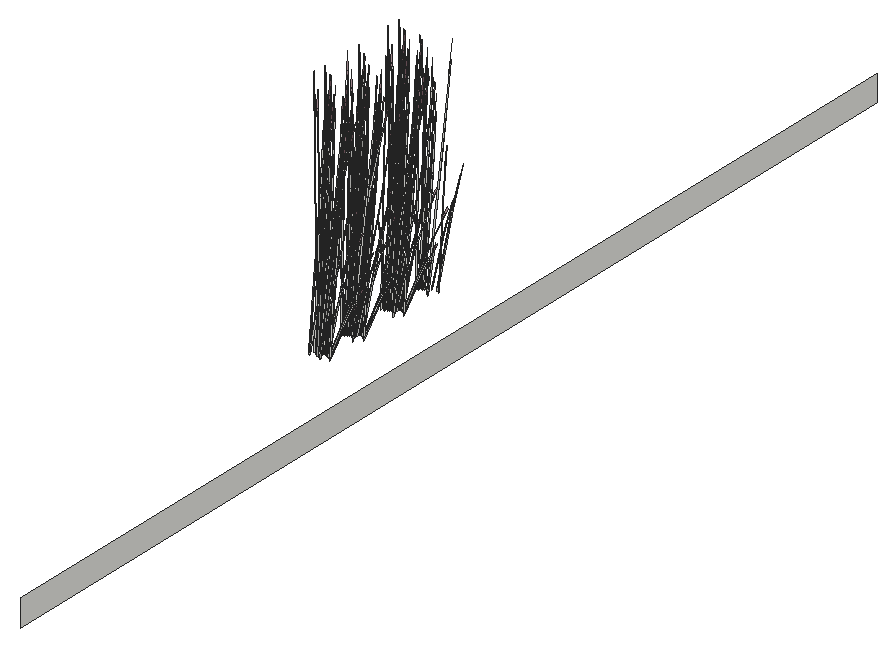
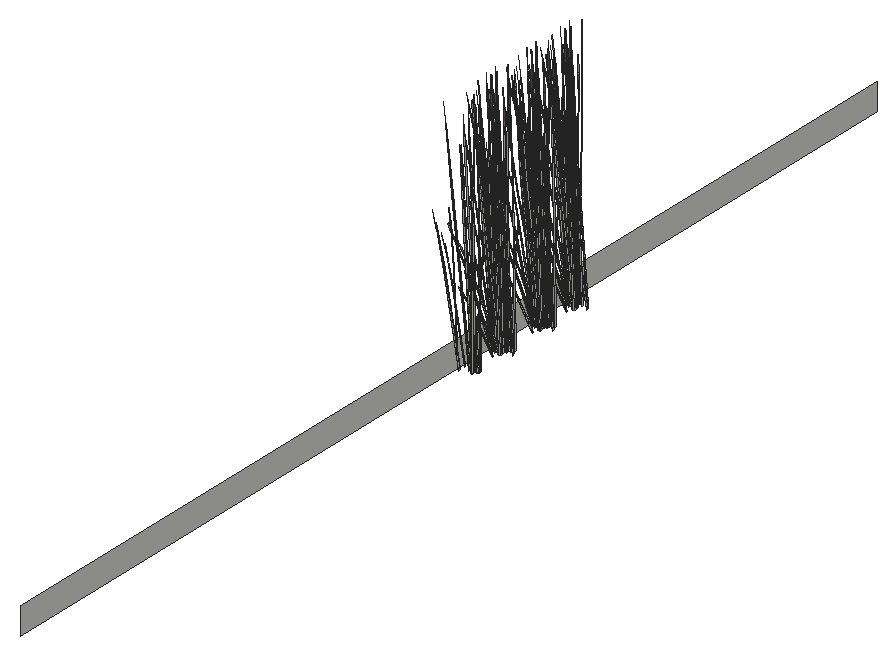
# SketchUp Ruby script. Lengths in inches.
U = 1.inch
M = Sketchup.active_model
def pt(a) = Geom::Point3d.new(a.map { |v| v * U })
def face(e, loops, mat)
  f = e.add_face(loops[0].map { |a| pt(a) })
  loops[1..].each { |l| e.add_face(l.map { |a| pt(a) }).erase! }
  f.material = f.back_material = mat if mat
  f
end
# faces: each face lists its corners as indices into pts; further lists are holes
def faces(e, pts, list, mat = nil) = list.each { |f| face(e, (f[0].is_a?(Array) ? f : [f]).map { |l| l.map { |i| pts[i] } }, mat) }
# xy, xz, yz: faces in a plane at the given z, y or x. An outline is a flat list of corners, or four numbers for a rectangle; further outlines are holes
def ring(l) = l.size == 4 ? [[l[0], l[1]], [l[2], l[1]], [l[2], l[3]], [l[0], l[3]]] : l.each_slice(2).to_a
def flat(e, list, mat, &to3) = list.each { |f| face(e, (f[0].is_a?(Array) ? f : [f]).map { |l| ring(l).map { |u, v| to3.(u, v) } }, mat) }
def xy(e, z, list, mat = nil) = flat(e, list, mat) { |x, y| [x, y, z] }
def xz(e, y, list, mat = nil) = flat(e, list, mat) { |x, z| [x, y, z] }
def yz(e, x, list, mat = nil) = flat(e, list, mat) { |y, z| [x, y, z] }
def lines(e, pts, list) = list.each { |a, b| e.add_line(pt(pts[a]), pt(pts[b])) }
# prism: a flat outline (further loops are holes) pulled along v
def prism(e, loops, v, mat = nil)
  f = face(e, loops, mat); d = Geom::Vector3d.new(v.map { |x| x * U })
  f.pushpull(f.normal.samedirection?(d) ? d.length : -d.length)
end
def box(e, o, s, mat = nil) = prism(e, [[o, [o[0] + s[0], o[1], o[2]], [o[0] + s[0], o[1] + s[1], o[2]], [o[0], o[1] + s[1], o[2]]]], [0, 0, s[2]], mat)
def at(x, y, z, deg = 0) = Geom::Transformation.translation(pt([x, y, z])) * Geom::Transformation.rotation(ORIGIN, Z_AXIS, deg.degrees)
def axes(o, x, y, z) = Geom::Transformation.new([*x, 0, *y, 0, *z, 0, *pt(o).to_a, 1])
def part(name) = M.definitions.add(name)
# library, detail: a bought-in or finely detailed component or shape, given as its bounding box
def library(name, o, s) = part(name).tap { |d| box(d.entities, o, s) }
def detail(e, o, s) = box(e.add_group.entities, o, s)
def put(e, d, t, mat = nil) = e.add_instance(d, t).tap { |i| i.material = mat if mat }
def group(e, t, mat = nil) = e.add_group.tap { |g| g.transformation = t; g.material = mat if mat }.entities
root = M.entities
M.materials.add("LightPink_Translucent").color = [144, 107, 117]
M.materials["LightPink_Translucent"].alpha = 0.75
c1 = part("blade")
p = [[2.15,0.21,22],[0,0.17,0],[0.09,0.45,0],[2.18,0.31,22],[2.29,0.31,22],[0.38,0.45,0],
  [2.48,0.24,33],[2.49,0.24,33],[2.48,0.22,33]]
faces(c1.entities,p,[[0,1,2,3],[4,5,2,3],[6,3,4,7],[8,0,3,6]])
c2 = part("seeds")
p = [[0.3,-0.1,1.38],[-0.01,-0.03,1.59],[-0.01,-0.03,0.03],[0.14,-0.07,-0.07],[0.29,-0.03,3],[0.15,0.01,3.11]]
faces(c2.entities,p,[[0,1,2,3],[1,0,4,5]],"LightPink_Translucent")
c3 = part("blade with seeds")
put(c3.entities,c1,at(0,0,0))
put(c3.entities,c2,axes([2.4,0.25,30.99],[1.5799,-0.05474,1.17369],[-0.12525,1.92788,0.29478],[-0.07173,-0.02425,1.56792]))
yz(root,346,[[268,42,508,48]])
put(root,c3,axes([335.24,364.91,50.1],[0.31568,-0.39156,0],[0.52815,0.21836,-0.456],[0.12029,0.04973,1.44655]))
put(root,c3,axes([336.49,366.46,49.75],[-0.3252,0.04689,1.25103],[-0.05176,-0.37326,0.07161],[0.22777,-0.0565,0.71188]))
put(root,c3,axes([337.08,366.125,50],[-0.31304,-0.24986,-0.05733],[0.34284,-0.22894,-0.25992],[0.09714,-0.01612,0.85731]))
put(root,c3,axes([334.21,366.16,49.95],[0,-0.45213,0],[0.63136,0,0],[0,0,1.58567]))
put(root,c3,axes([334.97,365.11,50.19],[-0.47255,-0.19538,0.43871],[0.28245,-0.35034,0],[0.10763,0.0445,1.3917]))
put(root,c3,axes([333.91,365.87,50.09],[-0.41865,0.35461,0.40429],[-0.49737,-0.31303,0.15865],[0.10093,-0.03539,1.40366]))
put(root,c3,axes([333.18,365.29,50.1875],[-0.14586,0.38834,0.15589],[-0.53375,-0.1099,0.31002],[0.0922,-0.00189,1.41735]))
put(root,c3,axes([332.96,365.6,49.41],[-0.49699,0.15644,1.13921],[-0.15819,-0.44887,0.44265],[0.30518,0.00747,1.29573]))
put(root,c3,axes([334.29,365.72,50.3125],[0.09741,-0.34873,0.12794],[0.4759,0.06053,-0.36534],[0.08661,0.03581,1.11991]))
put(root,c3,axes([336.84,366.21,49.32],[-0.02639,-0.05932,1.55816],[0.18302,-0.34702,-0.23804],[0.18462,-0.00499,0.26541]))
put(root,c3,axes([334.09,365.8125,50.4],[-0.30332,-0.32798,0.39531],[0.45944,-0.23096,-0.19025],[0.09816,0.04058,1.26923]))
put(root,c3,axes([334.25,365.83,50.36],[0.50979,-0.25942,-0.25709],[0.339,0.36656,-0.44182],[0.12578,0.03723,1.41118]))
put(root,c3,axes([335.53,365.14,49.78],[0.47255,0.19538,-0.43871],[-0.28245,0.35034,0],[0.10763,0.0445,1.3917]))
put(root,c3,axes([334.63,366.26,49.95],[0.56491,0,0],[0,0.40454,0],[0,0,1.5764]))
put(root,c3,axes([334.79,365.31,50.1875],[-0.54257,0.10371,0.15589],[-0.13397,-0.38597,0.31002],[0.04839,0.05624,1.41735]))
put(root,c3,axes([335.4,365.29,49.79],[0.11861,0.34048,-0.27372],[-0.47106,0.09668,0.27372],[0.09497,0.03926,1.22797]))
put(root,c3,axes([334.45,366.05,50.1],[-0.63817,-0.08233,0.43472],[0.12987,-0.46497,0.17059],[0.09326,0.0449,1.50931]))
put(root,c3,axes([334.56,367.15,49.93],[0.53009,-0.13258,-0.16963],[0.18627,0.38191,0.00007],[0.05851,-0.01465,1.53656]))
put(root,c3,axes([334.62,366.43,49.96],[0.35245,0.2524,0],[-0.35245,0.2524,0],[0,0,1.49564]))
put(root,c3,axes([335.58,366.32,50.1875],[-0.39671,-0.28463,0.15589],[0.39978,-0.27607,0.31002],[-0.04381,0.05813,1.41735]))
put(root,c3,axes([334.84,365.89,49.82],[0.52523,0.06406,-0.55095],[-0.11084,0.39517,-0.1446],[0.15674,0.04788,1.21613]))
put(root,c3,axes([334.62,366.14,50.4],[0.24498,-0.3521,0.39531],[0.50902,0.16945,-0.19025],[0,0.08116,1.26923]))
put(root,c3,axes([334.52,366.34,50.03],[0,0.45191,-0.04981],[-0.63136,0,0],[0,0.0142,1.58489]))
put(root,c3,axes([334.57,366.02,49.95],[0.30332,0.32798,-0.39531],[-0.45944,0.23096,0.19025],[0.09816,0.04058,1.26923]))
put(root,c3,axes([335.9,366.33,50.19],[0,-0.39075,0.43871],[0.56491,0,0],[0,0.089,1.3917]))
put(root,c3,axes([334.83,366.22,50.3125],[0.47043,-0.11396,0.12794],[0.16474,0.32541,-0.36534],[0,0.07162,1.11991]))
put(root,c3,axes([336.58,367.01,50.29],[-0.1216,-0.0961,1.26356],[0.15822,-0.31792,-0.27174],[0.24603,0.04307,0.54024]))
put(root,c3,axes([334.4,367.36,49.95],[0.50902,0.17543,0],[-0.24498,0.36452,0],[0,0,1.54589]))
put(root,c3,axes([334.22,367.21,50.02],[0.21952,0.44891,-0.05313],[-0.62724,0.1573,0],[0.00767,0.01568,1.52132]))
put(root,c3,axes([336.29,366.4,50.1],[0.63136,0,0],[0,0.43672,-0.456],[0,0.09947,1.44655]))
put(root,c3,axes([336.03,366.625,49.94],[-0.63105,-0.00312,-0.04397],[0,-0.43672,0.44129],[-0.01983,0.09942,1.3992]))
put(root,c3,axes([334.67,366.24,50.36],[0.56863,0.18645,-0.25709],[-0.2738,0.39352,-0.44182],[0.01787,0.09662,1.41118]))
put(root,c3,axes([335.9,366.6875,49.79],[-0.35245,0.2438,-0.27372],[-0.35245,-0.2438,0.27372],[0,0.07853,1.22797]))
put(root,c3,axes([336.15,366.7,49.78],[0,0.39075,-0.43871],[-0.56491,0,0],[0,0.089,1.3917]))
put(root,c3,axes([335.51,367.92,49.32],[0.03679,-0.05641,1.55816],[0.46313,-0.16615,-0.23804],[0.14041,0.08599,0.26541]))
put(root,c3,axes([334.9,366.64,49.85],[0.18514,0.35777,-0.61156],[-0.53331,0.12885,-0.16051],[0.02046,0.12115,1.3499]))
put(root,c3,axes([335.47,368.02,50.36],[-0.32378,-0.01225,0.92831],[0.21383,-0.26028,0.51254],[0.12791,0.09247,0.72818]))
put(root,c3,axes([334.42,367.39,50.29],[0.00891,-0.12953,1.26356],[0.4258,-0.14469,-0.27174],[0.13144,0.15503,0.54024]))
put(root,c3,axes([334.77,373.97,50.29],[-0.14352,0.07909,1.26356],[-0.42983,-0.13843,-0.27174],[0.07968,-0.17216,0.54024]))
put(root,c3,axes([335.77,374.21,49.32],[-0.07557,-0.03078,1.55816],[-0.19412,-0.34391,-0.23804],[0.13095,-0.09333,0.26541]))
put(root,c3,axes([332.92,374.28,50.1],[-0.31568,-0.39156,0],[0.52815,-0.21836,-0.456],[0.12029,-0.04973,1.44655]))
put(root,c3,axes([333.35,374.22,49.78],[0.47255,-0.19538,-0.43871],[0.28245,0.35034,0],[0.10763,-0.0445,1.3917]))
put(root,c3,axes([336.15,374.9,50.29],[-0.18038,-0.01157,1.26356],[-0.18479,-0.31048,-0.27174],[0.22159,-0.08783,0.54024]))
put(root,c3,axes([333.91,375.02,49.82],[0.34009,-0.2937,-0.55095],[0.42248,0.26632,-0.1446],[0.13628,-0.07327,1.21613]))
put(root,c3,axes([333.54,375.36,50.36],[-0.05884,-0.44587,-0.25709],[0.6128,-0.02696,-0.44182],[0.10791,-0.05939,1.41118]))
put(root,c3,axes([333.46,374.375,49.79],[0.47106,0.09668,-0.27372],[-0.11861,0.34048,0.27372],[0.09497,-0.03926,1.22797]))
put(root,c3,axes([333.62,375.71,50.15],[0.56891,0.18939,0.21263],[-0.2738,0.39352,0.44182],[0,-0.09071,1.41855]))
put(root,c3,axes([333.44,375.45,50.4],[-0.54829,0.02412,0.39531],[-0.04958,-0.40041,-0.19025],[0.09816,-0.04058,1.26923]))
put(root,c3,axes([335.24,374.38,50.1],[0.31568,-0.39156,0],[0.52815,0.21836,-0.456],[0.12029,0.04973,1.44655]))
put(root,c3,axes([336.49,375.93,49.75],[-0.3252,0.04689,1.25103],[-0.05176,-0.37326,0.07161],[0.22777,-0.0565,0.71188]))
put(root,c3,axes([337.08,375.6,50],[-0.31304,-0.24986,-0.05733],[0.34284,-0.22894,-0.25992],[0.09714,-0.01612,0.85731]))
put(root,c3,axes([334.21,375.63,49.95],[0,-0.45213,0],[0.63136,0,0],[0,0,1.58567]))
put(root,c3,axes([334.97,374.59,50.19],[-0.47255,-0.19538,0.43871],[0.28245,-0.35034,0],[0.10763,0.0445,1.3917]))
put(root,c3,axes([333.91,375.35,50.09],[-0.41865,0.35461,0.40429],[-0.49737,-0.31303,0.15865],[0.10093,-0.03539,1.40366]))
put(root,c3,axes([333.18,374.76,50.1875],[-0.14586,0.38834,0.15589],[-0.53375,-0.1099,0.31002],[0.0922,-0.00189,1.41735]))
put(root,c3,axes([332.96,375.07,49.41],[-0.49699,0.15644,1.13921],[-0.15819,-0.44887,0.44265],[0.30518,0.00747,1.29573]))
put(root,c3,axes([334.29,375.19,50.3125],[0.09741,-0.34873,0.12794],[0.4759,0.06053,-0.36534],[0.08661,0.03581,1.11991]))
put(root,c3,axes([336.84,375.68,49.32],[-0.02639,-0.05932,1.55816],[0.18302,-0.34702,-0.23804],[0.18462,-0.00499,0.26541]))
put(root,c3,axes([334.09,375.28,50.4],[-0.30332,-0.32798,0.39531],[0.45944,-0.23096,-0.19025],[0.09816,0.04058,1.26923]))
put(root,c3,axes([334.25,375.31,50.36],[0.50979,-0.25942,-0.25709],[0.339,0.36656,-0.44182],[0.12578,0.03723,1.41118]))
put(root,c3,axes([335.53,374.62,49.78],[0.47255,0.19538,-0.43871],[-0.28245,0.35034,0],[0.10763,0.0445,1.3917]))
put(root,c3,axes([334.63,375.73,49.95],[0.56491,0,0],[0,0.40454,0],[0,0,1.5764]))
put(root,c3,axes([334.79,374.78,50.1875],[-0.54257,0.10371,0.15589],[-0.13397,-0.38597,0.31002],[0.04839,0.05624,1.41735]))
put(root,c3,axes([335.4,374.76,49.79],[0.11861,0.34048,-0.27372],[-0.47106,0.09668,0.27372],[0.09497,0.03926,1.22797]))
put(root,c3,axes([334.45,375.53,50.1],[-0.63817,-0.08233,0.43472],[0.12987,-0.46497,0.17059],[0.09326,0.0449,1.50931]))
put(root,c3,axes([334.56,376.625,49.93],[0.53009,-0.13258,-0.16963],[0.18627,0.38191,0.00007],[0.05851,-0.01465,1.53656]))
put(root,c3,axes([334.62,375.9,49.96],[0.35245,0.2524,0],[-0.35245,0.2524,0],[0,0,1.49564]))
put(root,c3,axes([335.58,375.79,50.1875],[-0.39671,-0.28463,0.15589],[0.39978,-0.27607,0.31002],[-0.04381,0.05813,1.41735]))
put(root,c3,axes([334.84,375.36,49.82],[0.52523,0.06406,-0.55095],[-0.11084,0.39517,-0.1446],[0.15674,0.04788,1.21613]))
put(root,c3,axes([334.62,375.61,50.4],[0.24498,-0.3521,0.39531],[0.50902,0.16945,-0.19025],[0,0.08116,1.26923]))
put(root,c3,axes([334.52,375.8125,50.03],[0,0.45191,-0.04981],[-0.63136,0,0],[0,0.0142,1.58489]))
put(root,c3,axes([334.57,375.49,49.95],[0.30332,0.32798,-0.39531],[-0.45944,0.23096,0.19025],[0.09816,0.04058,1.26923]))
put(root,c3,axes([335.9,375.81,50.19],[0,-0.39075,0.43871],[0.56491,0,0],[0,0.089,1.3917]))
put(root,c3,axes([334.83,375.69,50.3125],[0.47043,-0.11396,0.12794],[0.16474,0.32541,-0.36534],[0,0.07162,1.11991]))
put(root,c3,axes([336.58,376.48,50.29],[-0.1216,-0.0961,1.26356],[0.15822,-0.31792,-0.27174],[0.24603,0.04307,0.54024]))
put(root,c3,axes([334.4,376.83,49.95],[0.50902,0.17543,0],[-0.24498,0.36452,0],[0,0,1.54589]))
put(root,c3,axes([334.22,376.68,50.02],[0.21952,0.44891,-0.05313],[-0.62724,0.1573,0],[0.00767,0.01568,1.52132]))
put(root,c3,axes([336.29,375.87,50.1],[0.63136,0,0],[0,0.43672,-0.456],[0,0.09947,1.44655]))
put(root,c3,axes([336.03,376.1,49.94],[-0.63105,-0.00312,-0.04397],[0,-0.43672,0.44129],[-0.01983,0.09942,1.3992]))
put(root,c3,axes([334.67,375.72,50.36],[0.56863,0.18645,-0.25709],[-0.2738,0.39352,-0.44182],[0.01787,0.09662,1.41118]))
put(root,c3,axes([335.9,376.16,49.79],[-0.35245,0.2438,-0.27372],[-0.35245,-0.2438,0.27372],[0,0.07853,1.22797]))
put(root,c3,axes([336.15,376.17,49.78],[0,0.39075,-0.43871],[-0.56491,0,0],[0,0.089,1.3917]))
put(root,c3,axes([335.51,377.4,49.32],[0.03679,-0.05641,1.55816],[0.46313,-0.16615,-0.23804],[0.14041,0.08599,0.26541]))
put(root,c3,axes([334.9,376.11,49.85],[0.18514,0.35777,-0.61156],[-0.53331,0.12885,-0.16051],[0.02046,0.12115,1.3499]))
put(root,c3,axes([335.47,377.49,50.36],[-0.32378,-0.01225,0.92831],[0.21383,-0.26028,0.51254],[0.12791,0.09247,0.72818]))
put(root,c3,axes([334.42,376.86,50.29],[0.00891,-0.12953,1.26356],[0.4258,-0.14469,-0.27174],[0.13144,0.15503,0.54024]))
put(root,c3,axes([334.77,385.27,50.29],[-0.14352,0.07909,1.26356],[-0.42983,-0.13843,-0.27174],[0.07968,-0.17216,0.54024]))
put(root,c3,axes([335.77,385.52,49.32],[-0.07557,-0.03078,1.55816],[-0.19412,-0.34391,-0.23804],[0.13095,-0.09333,0.26541]))
put(root,c3,axes([332.92,385.59,50.1],[-0.31568,-0.39156,0],[0.52815,-0.21836,-0.456],[0.12029,-0.04973,1.44655]))
put(root,c3,axes([333.35,385.53,49.78],[0.47255,-0.19538,-0.43871],[0.28245,0.35034,0],[0.10763,-0.0445,1.3917]))
put(root,c3,axes([336.15,386.21,50.29],[-0.18038,-0.01157,1.26356],[-0.18479,-0.31048,-0.27174],[0.22159,-0.08783,0.54024]))
put(root,c3,axes([333.91,386.33,49.82],[0.34009,-0.2937,-0.55095],[0.42248,0.26632,-0.1446],[0.13628,-0.07327,1.21613]))
put(root,c3,axes([333.54,386.67,50.36],[-0.05884,-0.44587,-0.25709],[0.6128,-0.02696,-0.44182],[0.10791,-0.05939,1.41118]))
put(root,c3,axes([333.46,385.68,49.79],[0.47106,0.09668,-0.27372],[-0.11861,0.34048,0.27372],[0.09497,-0.03926,1.22797]))
put(root,c3,axes([333.62,387.02,50.15],[0.56891,0.18939,0.21263],[-0.2738,0.39352,0.44182],[0,-0.09071,1.41855]))
put(root,c3,axes([333.44,386.76,50.4],[-0.54829,0.02412,0.39531],[-0.04958,-0.40041,-0.19025],[0.09816,-0.04058,1.26923]))
put(root,c3,axes([335.24,385.69,50.1],[0.31568,-0.39156,0],[0.52815,0.21836,-0.456],[0.12029,0.04973,1.44655]))
put(root,c3,axes([336.49,387.24,49.75],[-0.3252,0.04689,1.25103],[-0.05176,-0.37326,0.07161],[0.22777,-0.0565,0.71188]))
put(root,c3,axes([337.08,386.91,50],[-0.31304,-0.24986,-0.05733],[0.34284,-0.22894,-0.25992],[0.09714,-0.01612,0.85731]))
put(root,c3,axes([334.21,386.9375,49.95],[0,-0.45213,0],[0.63136,0,0],[0,0,1.58567]))
put(root,c3,axes([334.97,385.89,50.19],[-0.47255,-0.19538,0.43871],[0.28245,-0.35034,0],[0.10763,0.0445,1.3917]))
put(root,c3,axes([333.91,386.65,50.09],[-0.41865,0.35461,0.40429],[-0.49737,-0.31303,0.15865],[0.10093,-0.03539,1.40366]))
put(root,c3,axes([333.18,386.07,50.1875],[-0.14586,0.38834,0.15589],[-0.53375,-0.1099,0.31002],[0.0922,-0.00189,1.41735]))
put(root,c3,axes([332.96,386.38,49.41],[-0.49699,0.15644,1.13921],[-0.15819,-0.44887,0.44265],[0.30518,0.00747,1.29573]))
put(root,c3,axes([334.29,386.5,50.3125],[0.09741,-0.34873,0.12794],[0.4759,0.06053,-0.36534],[0.08661,0.03581,1.11991]))
put(root,c3,axes([336.84,386.99,49.32],[-0.02639,-0.05932,1.55816],[0.18302,-0.34702,-0.23804],[0.18462,-0.00499,0.26541]))
put(root,c3,axes([334.09,386.59,50.4],[-0.30332,-0.32798,0.39531],[0.45944,-0.23096,-0.19025],[0.09816,0.04058,1.26923]))
put(root,c3,axes([334.25,386.61,50.36],[0.50979,-0.25942,-0.25709],[0.339,0.36656,-0.44182],[0.12578,0.03723,1.41118]))
put(root,c3,axes([335.53,385.93,49.78],[0.47255,0.19538,-0.43871],[-0.28245,0.35034,0],[0.10763,0.0445,1.3917]))
put(root,c3,axes([334.63,387.04,49.95],[0.56491,0,0],[0,0.40454,0],[0,0,1.5764]))
put(root,c3,axes([334.79,386.09,50.1875],[-0.54257,0.10371,0.15589],[-0.13397,-0.38597,0.31002],[0.04839,0.05624,1.41735]))
put(root,c3,axes([335.4,386.07,49.79],[0.11861,0.34048,-0.27372],[-0.47106,0.09668,0.27372],[0.09497,0.03926,1.22797]))
put(root,c3,axes([334.45,386.83,50.1],[-0.63817,-0.08233,0.43472],[0.12987,-0.46497,0.17059],[0.09326,0.0449,1.50931]))
put(root,c3,axes([334.56,387.93,49.93],[0.53009,-0.13258,-0.16963],[0.18627,0.38191,0.00007],[0.05851,-0.01465,1.53656]))
put(root,c3,axes([334.62,387.21,49.96],[0.35245,0.2524,0],[-0.35245,0.2524,0],[0,0,1.49564]))
put(root,c3,axes([335.58,387.1,50.1875],[-0.39671,-0.28463,0.15589],[0.39978,-0.27607,0.31002],[-0.04381,0.05813,1.41735]))
put(root,c3,axes([334.84,386.67,49.82],[0.52523,0.06406,-0.55095],[-0.11084,0.39517,-0.1446],[0.15674,0.04788,1.21613]))
put(root,c3,axes([334.62,386.92,50.4],[0.24498,-0.3521,0.39531],[0.50902,0.16945,-0.19025],[0,0.08116,1.26923]))
put(root,c3,axes([334.52,387.12,50.03],[0,0.45191,-0.04981],[-0.63136,0,0],[0,0.0142,1.58489]))
put(root,c3,axes([334.57,386.8,49.95],[0.30332,0.32798,-0.39531],[-0.45944,0.23096,0.19025],[0.09816,0.04058,1.26923]))
put(root,c3,axes([335.9,387.11,50.19],[0,-0.39075,0.43871],[0.56491,0,0],[0,0.089,1.3917]))
put(root,c3,axes([334.83,387,50.3125],[0.47043,-0.11396,0.12794],[0.16474,0.32541,-0.36534],[0,0.07162,1.11991]))
put(root,c3,axes([336.58,387.79,50.29],[-0.1216,-0.0961,1.26356],[0.15822,-0.31792,-0.27174],[0.24603,0.04307,0.54024]))
put(root,c3,axes([334.4,388.14,49.95],[0.50902,0.17543,0],[-0.24498,0.36452,0],[0,0,1.54589]))
put(root,c3,axes([334.22,387.99,50.02],[0.21952,0.44891,-0.05313],[-0.62724,0.1573,0],[0.00767,0.01568,1.52132]))
put(root,c3,axes([336.29,387.18,50.1],[0.63136,0,0],[0,0.43672,-0.456],[0,0.09947,1.44655]))
put(root,c3,axes([336.03,387.41,49.94],[-0.63105,-0.00312,-0.04397],[0,-0.43672,0.44129],[-0.01983,0.09942,1.3992]))
put(root,c3,axes([334.67,387.02,50.36],[0.56863,0.18645,-0.25709],[-0.2738,0.39352,-0.44182],[0.01787,0.09662,1.41118]))
put(root,c3,axes([335.9,387.47,49.79],[-0.35245,0.2438,-0.27372],[-0.35245,-0.2438,0.27372],[0,0.07853,1.22797]))
put(root,c3,axes([336.15,387.48,49.78],[0,0.39075,-0.43871],[-0.56491,0,0],[0,0.089,1.3917]))
put(root,c3,axes([335.51,388.7,49.32],[0.03679,-0.05641,1.55816],[0.46313,-0.16615,-0.23804],[0.14041,0.08599,0.26541]))
put(root,c3,axes([334.9,387.42,49.85],[0.18514,0.35777,-0.61156],[-0.53331,0.12885,-0.16051],[0.02046,0.12115,1.3499]))
put(root,c3,axes([335.47,388.8,50.36],[-0.32378,-0.01225,0.92831],[0.21383,-0.26028,0.51254],[0.12791,0.09247,0.72818]))
put(root,c3,axes([334.42,388.17,50.29],[0.00891,-0.12953,1.26356],[0.4258,-0.14469,-0.27174],[0.13144,0.15503,0.54024]))
put(root,c3,axes([334.77,394.96,50.29],[-0.14352,0.07909,1.26356],[-0.42983,-0.13843,-0.27174],[0.07968,-0.17216,0.54024]))
put(root,c3,axes([335.77,395.2,49.32],[-0.07557,-0.03078,1.55816],[-0.19412,-0.34391,-0.23804],[0.13095,-0.09333,0.26541]))
put(root,c3,axes([332.92,395.27,50.1],[-0.31568,-0.39156,0],[0.52815,-0.21836,-0.456],[0.12029,-0.04973,1.44655]))
put(root,c3,axes([333.35,395.21,49.78],[0.47255,-0.19538,-0.43871],[0.28245,0.35034,0],[0.10763,-0.0445,1.3917]))
put(root,c3,axes([336.15,395.89,50.29],[-0.18038,-0.01157,1.26356],[-0.18479,-0.31048,-0.27174],[0.22159,-0.08783,0.54024]))
put(root,c3,axes([333.91,396.01,49.82],[0.34009,-0.2937,-0.55095],[0.42248,0.26632,-0.1446],[0.13628,-0.07327,1.21613]))
put(root,c3,axes([333.54,396.35,50.36],[-0.05884,-0.44587,-0.25709],[0.6128,-0.02696,-0.44182],[0.10791,-0.05939,1.41118]))
put(root,c3,axes([333.46,395.37,49.79],[0.47106,0.09668,-0.27372],[-0.11861,0.34048,0.27372],[0.09497,-0.03926,1.22797]))
put(root,c3,axes([333.62,396.7,50.15],[0.56891,0.18939,0.21263],[-0.2738,0.39352,0.44182],[0,-0.09071,1.41855]))
put(root,c3,axes([333.44,396.4375,50.4],[-0.54829,0.02412,0.39531],[-0.04958,-0.40041,-0.19025],[0.09816,-0.04058,1.26923]))
put(root,c3,axes([335.24,395.37,50.1],[0.31568,-0.39156,0],[0.52815,0.21836,-0.456],[0.12029,0.04973,1.44655]))
put(root,c3,axes([336.49,396.92,49.75],[-0.3252,0.04689,1.25103],[-0.05176,-0.37326,0.07161],[0.22777,-0.0565,0.71188]))
put(root,c3,axes([337.08,396.59,50],[-0.31304,-0.24986,-0.05733],[0.34284,-0.22894,-0.25992],[0.09714,-0.01612,0.85731]))
